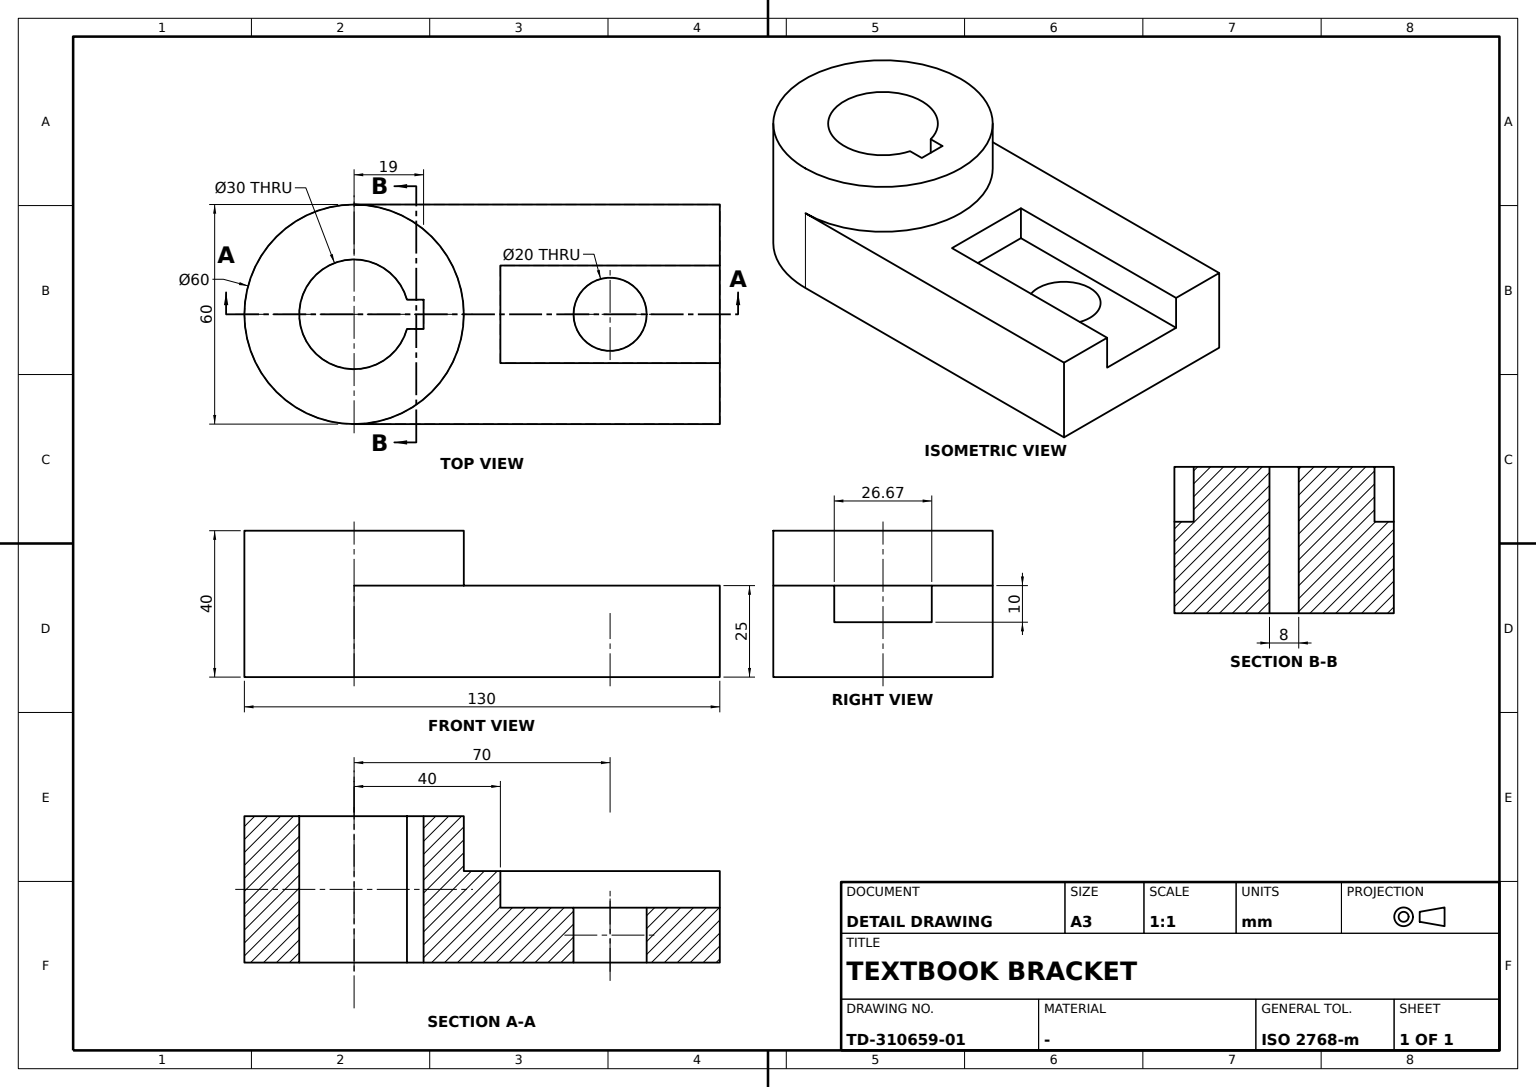
ISO-10303-21;
HEADER;
FILE_DESCRIPTION((''),'2;1');
FILE_NAME('','',(''),(''),'','','');
FILE_SCHEMA(('AUTOMOTIVE_DESIGN'));
ENDSEC;
DATA;
#1=APPLICATION_CONTEXT('');
#2=PRODUCT_CONTEXT('',#1,'mechanical');
#3=PRODUCT('','','',(#2));
#4=PRODUCT_DEFINITION_FORMATION('','',#3);
#5=PRODUCT_DEFINITION_CONTEXT('',#1,'design');
#6=PRODUCT_DEFINITION('','',#4,#5);
#7=PRODUCT_DEFINITION_SHAPE('','',#6);
#8=(LENGTH_UNIT()NAMED_UNIT(*)SI_UNIT(.MILLI.,.METRE.));
#9=(NAMED_UNIT(*)PLANE_ANGLE_UNIT()SI_UNIT($,.RADIAN.));
#10=(NAMED_UNIT(*)SI_UNIT($,.STERADIAN.)SOLID_ANGLE_UNIT());
#11=UNCERTAINTY_MEASURE_WITH_UNIT(LENGTH_MEASURE(1.E-05),#8,'distance_accuracy_value','');
#12=(GEOMETRIC_REPRESENTATION_CONTEXT(3)GLOBAL_UNCERTAINTY_ASSIGNED_CONTEXT((#11))GLOBAL_UNIT_ASSIGNED_CONTEXT((#8,#9,#10))REPRESENTATION_CONTEXT('',''));
#13=CARTESIAN_POINT('',(-4.,14.456832,0.));
#14=VERTEX_POINT('',#13);
#15=CARTESIAN_POINT('',(4.,14.456832,0.));
#16=VERTEX_POINT('',#15);
#17=CARTESIAN_POINT('',(0.,0.,0.));
#18=DIRECTION('',(0.,0.,1.));
#19=DIRECTION('',(0.,1.,0.));
#20=AXIS2_PLACEMENT_3D('',#17,#18,#19);
#21=CIRCLE('',#20,15.);
#22=EDGE_CURVE('',#14,#16,#21,.T.);
#23=ORIENTED_EDGE('',*,*,#22,.T.);
#24=CARTESIAN_POINT('',(4.,19.,0.));
#25=VERTEX_POINT('',#24);
#26=CARTESIAN_POINT('',(4.,16.728416,0.));
#27=VECTOR('',#19,1000.);
#28=LINE('',#26,#27);
#29=EDGE_CURVE('',#16,#25,#28,.T.);
#30=ORIENTED_EDGE('',*,*,#29,.T.);
#31=CARTESIAN_POINT('',(-4.,19.,0.));
#32=VERTEX_POINT('',#31);
#33=CARTESIAN_POINT('',(0.,19.,0.));
#34=DIRECTION('',(-1.,0.,0.));
#35=VECTOR('',#34,1000.);
#36=LINE('',#33,#35);
#37=EDGE_CURVE('',#25,#32,#36,.T.);
#38=ORIENTED_EDGE('',*,*,#37,.T.);
#39=CARTESIAN_POINT('',(-4.,16.728416,0.));
#40=DIRECTION('',(0.,-1.,0.));
#41=VECTOR('',#40,1000.);
#42=LINE('',#39,#41);
#43=EDGE_CURVE('',#32,#14,#42,.T.);
#44=ORIENTED_EDGE('',*,*,#43,.T.);
#45=EDGE_LOOP('',(#23,#30,#38,#44));
#46=FACE_BOUND('',#45,.T.);
#47=CARTESIAN_POINT('',(-30.,100.,0.));
#48=VERTEX_POINT('',#47);
#49=CARTESIAN_POINT('',(-30.,0.,0.));
#50=VERTEX_POINT('',#49);
#51=CARTESIAN_POINT('',(-30.,50.,0.));
#52=LINE('',#51,#41);
#53=EDGE_CURVE('',#48,#50,#52,.T.);
#54=ORIENTED_EDGE('',*,*,#53,.F.);
#55=CARTESIAN_POINT('',(30.,100.,0.));
#56=VERTEX_POINT('',#55);
#57=CARTESIAN_POINT('',(0.,100.,0.));
#58=DIRECTION('',(1.,0.,0.));
#59=VECTOR('',#58,1000.);
#60=LINE('',#57,#59);
#61=EDGE_CURVE('',#48,#56,#60,.T.);
#62=ORIENTED_EDGE('',*,*,#61,.T.);
#63=CARTESIAN_POINT('',(30.,0.,0.));
#64=VERTEX_POINT('',#63);
#65=CARTESIAN_POINT('',(30.,50.,0.));
#66=LINE('',#65,#27);
#67=EDGE_CURVE('',#64,#56,#66,.T.);
#68=ORIENTED_EDGE('',*,*,#67,.F.);
#69=CIRCLE('',#20,30.);
#70=EDGE_CURVE('',#50,#64,#69,.T.);
#71=ORIENTED_EDGE('',*,*,#70,.F.);
#72=EDGE_LOOP('',(#54,#62,#68,#71));
#73=FACE_OUTER_BOUND('',#72,.T.);
#74=CARTESIAN_POINT('',(0.,80.,0.));
#75=VERTEX_POINT('',#74);
#76=CARTESIAN_POINT('',(0.,60.,0.));
#77=VERTEX_POINT('',#76);
#78=CARTESIAN_POINT('',(0.,70.,0.));
#79=AXIS2_PLACEMENT_3D('',#78,#18,#19);
#80=CIRCLE('',#79,10.);
#81=EDGE_CURVE('',#75,#77,#80,.T.);
#82=ORIENTED_EDGE('',*,*,#81,.T.);
#83=EDGE_CURVE('',#77,#75,#80,.T.);
#84=ORIENTED_EDGE('',*,*,#83,.T.);
#85=EDGE_LOOP('',(#82,#84));
#86=FACE_BOUND('',#85,.T.);
#87=PLANE('',#20);
#88=ADVANCED_FACE('',(#46,#73,#86),#87,.F.);
#89=CARTESIAN_POINT('',(-4.,14.456832,40.));
#90=VERTEX_POINT('',#89);
#91=CARTESIAN_POINT('',(4.,14.456832,40.));
#92=VERTEX_POINT('',#91);
#93=CARTESIAN_POINT('',(0.,0.,40.));
#94=AXIS2_PLACEMENT_3D('',#93,#18,#19);
#95=CIRCLE('',#94,15.);
#96=EDGE_CURVE('',#90,#92,#95,.T.);
#97=ORIENTED_EDGE('',*,*,#96,.T.);
#98=CARTESIAN_POINT('',(4.,14.456832,20.));
#99=VECTOR('',#18,1000.);
#100=LINE('',#98,#99);
#101=EDGE_CURVE('',#16,#92,#100,.T.);
#102=ORIENTED_EDGE('',*,*,#101,.F.);
#103=ORIENTED_EDGE('',*,*,#22,.F.);
#104=CARTESIAN_POINT('',(-4.,14.456832,20.));
#105=LINE('',#104,#99);
#106=EDGE_CURVE('',#14,#90,#105,.T.);
#107=ORIENTED_EDGE('',*,*,#106,.T.);
#108=EDGE_LOOP('',(#97,#102,#103,#107));
#109=FACE_OUTER_BOUND('',#108,.T.);
#110=CARTESIAN_POINT('',(0.,0.,20.));
#111=DIRECTION('',(0.,0.,-1.));
#112=AXIS2_PLACEMENT_3D('',#110,#111,#19);
#113=CYLINDRICAL_SURFACE('',#112,15.);
#114=ADVANCED_FACE('',(#109),#113,.F.);
#115=CARTESIAN_POINT('',(-4.,19.,40.));
#116=VERTEX_POINT('',#115);
#117=CARTESIAN_POINT('',(-4.,19.,20.));
#118=LINE('',#117,#99);
#119=EDGE_CURVE('',#32,#116,#118,.T.);
#120=ORIENTED_EDGE('',*,*,#119,.F.);
#121=ORIENTED_EDGE('',*,*,#37,.F.);
#122=CARTESIAN_POINT('',(4.,19.,40.));
#123=VERTEX_POINT('',#122);
#124=CARTESIAN_POINT('',(4.,19.,20.));
#125=LINE('',#124,#99);
#126=EDGE_CURVE('',#25,#123,#125,.T.);
#127=ORIENTED_EDGE('',*,*,#126,.T.);
#128=CARTESIAN_POINT('',(0.,19.,40.));
#129=LINE('',#128,#35);
#130=EDGE_CURVE('',#123,#116,#129,.T.);
#131=ORIENTED_EDGE('',*,*,#130,.T.);
#132=EDGE_LOOP('',(#120,#121,#127,#131));
#133=FACE_OUTER_BOUND('',#132,.T.);
#134=AXIS2_PLACEMENT_3D('',#31,#40,#58);
#135=PLANE('',#134);
#136=ADVANCED_FACE('',(#133),#135,.T.);
#137=CARTESIAN_POINT('',(0.,30.,25.));
#138=VERTEX_POINT('',#137);
#139=CARTESIAN_POINT('',(-30.,0.,25.));
#140=VERTEX_POINT('',#139);
#141=CARTESIAN_POINT('',(0.,0.,25.));
#142=AXIS2_PLACEMENT_3D('',#141,#18,#19);
#143=CIRCLE('',#142,30.);
#144=EDGE_CURVE('',#138,#140,#143,.T.);
#145=ORIENTED_EDGE('',*,*,#144,.F.);
#146=CARTESIAN_POINT('',(30.,0.,25.));
#147=VERTEX_POINT('',#146);
#148=EDGE_CURVE('',#147,#138,#143,.T.);
#149=ORIENTED_EDGE('',*,*,#148,.F.);
#150=CARTESIAN_POINT('',(30.,100.,25.));
#151=VERTEX_POINT('',#150);
#152=CARTESIAN_POINT('',(30.,50.,25.));
#153=LINE('',#152,#27);
#154=EDGE_CURVE('',#147,#151,#153,.T.);
#155=ORIENTED_EDGE('',*,*,#154,.T.);
#156=CARTESIAN_POINT('',(13.332727,100.,25.));
#157=VERTEX_POINT('',#156);
#158=CARTESIAN_POINT('',(21.666364,100.,25.));
#159=LINE('',#158,#59);
#160=EDGE_CURVE('',#157,#151,#159,.T.);
#161=ORIENTED_EDGE('',*,*,#160,.F.);
#162=CARTESIAN_POINT('',(13.332727,40.,25.));
#163=VERTEX_POINT('',#162);
#164=CARTESIAN_POINT('',(13.332727,70.,25.));
#165=LINE('',#164,#41);
#166=EDGE_CURVE('',#157,#163,#165,.T.);
#167=ORIENTED_EDGE('',*,*,#166,.T.);
#168=CARTESIAN_POINT('',(-13.332727,40.,25.));
#169=VERTEX_POINT('',#168);
#170=CARTESIAN_POINT('',(0.,40.,25.));
#171=LINE('',#170,#59);
#172=EDGE_CURVE('',#169,#163,#171,.T.);
#173=ORIENTED_EDGE('',*,*,#172,.F.);
#174=CARTESIAN_POINT('',(-13.332727,100.,25.));
#175=VERTEX_POINT('',#174);
#176=CARTESIAN_POINT('',(-13.332727,70.,25.));
#177=LINE('',#176,#41);
#178=EDGE_CURVE('',#175,#169,#177,.T.);
#179=ORIENTED_EDGE('',*,*,#178,.F.);
#180=CARTESIAN_POINT('',(-30.,100.,25.));
#181=VERTEX_POINT('',#180);
#182=CARTESIAN_POINT('',(-21.666364,100.,25.));
#183=LINE('',#182,#59);
#184=EDGE_CURVE('',#181,#175,#183,.T.);
#185=ORIENTED_EDGE('',*,*,#184,.F.);
#186=CARTESIAN_POINT('',(-30.,50.,25.));
#187=LINE('',#186,#41);
#188=EDGE_CURVE('',#181,#140,#187,.T.);
#189=ORIENTED_EDGE('',*,*,#188,.T.);
#190=EDGE_LOOP('',(#145,#149,#155,#161,#167,#173,#179,#185,#189));
#191=FACE_OUTER_BOUND('',#190,.T.);
#192=PLANE('',#142);
#193=ADVANCED_FACE('',(#191),#192,.T.);
#194=CARTESIAN_POINT('',(0.,80.,15.));
#195=VERTEX_POINT('',#194);
#196=CARTESIAN_POINT('',(0.,60.,15.));
#197=VERTEX_POINT('',#196);
#198=CARTESIAN_POINT('',(0.,70.,15.));
#199=AXIS2_PLACEMENT_3D('',#198,#111,#58);
#200=CIRCLE('',#199,10.);
#201=EDGE_CURVE('',#195,#197,#200,.T.);
#202=ORIENTED_EDGE('',*,*,#201,.T.);
#203=EDGE_CURVE('',#197,#195,#200,.T.);
#204=ORIENTED_EDGE('',*,*,#203,.T.);
#205=EDGE_LOOP('',(#202,#204));
#206=FACE_BOUND('',#205,.T.);
#207=CARTESIAN_POINT('',(-13.332727,100.,15.));
#208=VERTEX_POINT('',#207);
#209=CARTESIAN_POINT('',(-13.332727,40.,15.));
#210=VERTEX_POINT('',#209);
#211=CARTESIAN_POINT('',(-13.332727,70.,15.));
#212=LINE('',#211,#41);
#213=EDGE_CURVE('',#208,#210,#212,.T.);
#214=ORIENTED_EDGE('',*,*,#213,.T.);
#215=CARTESIAN_POINT('',(13.332727,40.,15.));
#216=VERTEX_POINT('',#215);
#217=CARTESIAN_POINT('',(0.,40.,15.));
#218=LINE('',#217,#35);
#219=EDGE_CURVE('',#216,#210,#218,.T.);
#220=ORIENTED_EDGE('',*,*,#219,.F.);
#221=CARTESIAN_POINT('',(13.332727,100.,15.));
#222=VERTEX_POINT('',#221);
#223=CARTESIAN_POINT('',(13.332727,70.,15.));
#224=LINE('',#223,#41);
#225=EDGE_CURVE('',#222,#216,#224,.T.);
#226=ORIENTED_EDGE('',*,*,#225,.F.);
#227=CARTESIAN_POINT('',(0.,100.,15.));
#228=LINE('',#227,#35);
#229=EDGE_CURVE('',#222,#208,#228,.T.);
#230=ORIENTED_EDGE('',*,*,#229,.T.);
#231=EDGE_LOOP('',(#214,#220,#226,#230));
#232=FACE_OUTER_BOUND('',#231,.T.);
#233=AXIS2_PLACEMENT_3D('',#207,#111,#58);
#234=PLANE('',#233);
#235=ADVANCED_FACE('',(#206,#232),#234,.F.);
#236=CARTESIAN_POINT('',(-30.,0.,40.));
#237=VERTEX_POINT('',#236);
#238=CARTESIAN_POINT('',(30.,0.,40.));
#239=VERTEX_POINT('',#238);
#240=CIRCLE('',#94,30.);
#241=EDGE_CURVE('',#237,#239,#240,.T.);
#242=ORIENTED_EDGE('',*,*,#241,.T.);
#243=CARTESIAN_POINT('',(0.,30.,40.));
#244=VERTEX_POINT('',#243);
#245=EDGE_CURVE('',#239,#244,#240,.T.);
#246=ORIENTED_EDGE('',*,*,#245,.T.);
#247=EDGE_CURVE('',#244,#237,#240,.T.);
#248=ORIENTED_EDGE('',*,*,#247,.T.);
#249=EDGE_LOOP('',(#242,#246,#248));
#250=FACE_OUTER_BOUND('',#249,.T.);
#251=CARTESIAN_POINT('',(-4.,16.728416,40.));
#252=LINE('',#251,#41);
#253=EDGE_CURVE('',#116,#90,#252,.T.);
#254=ORIENTED_EDGE('',*,*,#253,.F.);
#255=ORIENTED_EDGE('',*,*,#130,.F.);
#256=CARTESIAN_POINT('',(4.,16.728416,40.));
#257=LINE('',#256,#27);
#258=EDGE_CURVE('',#92,#123,#257,.T.);
#259=ORIENTED_EDGE('',*,*,#258,.F.);
#260=ORIENTED_EDGE('',*,*,#96,.F.);
#261=EDGE_LOOP('',(#254,#255,#259,#260));
#262=FACE_BOUND('',#261,.T.);
#263=PLANE('',#94);
#264=ADVANCED_FACE('',(#250,#262),#263,.T.);
#265=CARTESIAN_POINT('',(-13.332727,40.,20.));
#266=LINE('',#265,#99);
#267=EDGE_CURVE('',#210,#169,#266,.T.);
#268=ORIENTED_EDGE('',*,*,#267,.T.);
#269=ORIENTED_EDGE('',*,*,#172,.T.);
#270=CARTESIAN_POINT('',(13.332727,40.,20.));
#271=VECTOR('',#111,1000.);
#272=LINE('',#270,#271);
#273=EDGE_CURVE('',#163,#216,#272,.T.);
#274=ORIENTED_EDGE('',*,*,#273,.T.);
#275=ORIENTED_EDGE('',*,*,#219,.T.);
#276=EDGE_LOOP('',(#268,#269,#274,#275));
#277=FACE_OUTER_BOUND('',#276,.T.);
#278=CARTESIAN_POINT('',(0.,40.,0.));
#279=AXIS2_PLACEMENT_3D('',#278,#19,#34);
#280=PLANE('',#279);
#281=ADVANCED_FACE('',(#277),#280,.T.);
#282=ORIENTED_EDGE('',*,*,#53,.T.);
#283=CARTESIAN_POINT('',(-30.,0.,12.5));
#284=LINE('',#283,#99);
#285=EDGE_CURVE('',#50,#140,#284,.T.);
#286=ORIENTED_EDGE('',*,*,#285,.T.);
#287=ORIENTED_EDGE('',*,*,#188,.F.);
#288=CARTESIAN_POINT('',(-30.,100.,12.5));
#289=LINE('',#288,#99);
#290=EDGE_CURVE('',#48,#181,#289,.T.);
#291=ORIENTED_EDGE('',*,*,#290,.F.);
#292=EDGE_LOOP('',(#282,#286,#287,#291));
#293=FACE_OUTER_BOUND('',#292,.T.);
#294=AXIS2_PLACEMENT_3D('',#49,#58,#19);
#295=PLANE('',#294);
#296=ADVANCED_FACE('',(#293),#295,.F.);
#297=CARTESIAN_POINT('',(30.,0.,20.));
#298=LINE('',#297,#99);
#299=EDGE_CURVE('',#147,#239,#298,.T.);
#300=ORIENTED_EDGE('',*,*,#299,.F.);
#301=ORIENTED_EDGE('',*,*,#148,.T.);
#302=CARTESIAN_POINT('',(0.,30.,20.));
#303=LINE('',#302,#99);
#304=EDGE_CURVE('',#138,#244,#303,.T.);
#305=ORIENTED_EDGE('',*,*,#304,.T.);
#306=ORIENTED_EDGE('',*,*,#245,.F.);
#307=EDGE_LOOP('',(#300,#301,#305,#306));
#308=FACE_OUTER_BOUND('',#307,.T.);
#309=CYLINDRICAL_SURFACE('',#112,30.);
#310=ADVANCED_FACE('',(#308),#309,.T.);
#311=ORIENTED_EDGE('',*,*,#126,.F.);
#312=ORIENTED_EDGE('',*,*,#29,.F.);
#313=ORIENTED_EDGE('',*,*,#101,.T.);
#314=ORIENTED_EDGE('',*,*,#258,.T.);
#315=EDGE_LOOP('',(#311,#312,#313,#314));
#316=FACE_OUTER_BOUND('',#315,.T.);
#317=AXIS2_PLACEMENT_3D('',#24,#34,#40);
#318=PLANE('',#317);
#319=ADVANCED_FACE('',(#316),#318,.T.);
#320=CARTESIAN_POINT('',(30.,0.,12.5));
#321=LINE('',#320,#99);
#322=EDGE_CURVE('',#64,#147,#321,.T.);
#323=ORIENTED_EDGE('',*,*,#322,.F.);
#324=ORIENTED_EDGE('',*,*,#67,.T.);
#325=CARTESIAN_POINT('',(30.,100.,12.5));
#326=LINE('',#325,#99);
#327=EDGE_CURVE('',#56,#151,#326,.T.);
#328=ORIENTED_EDGE('',*,*,#327,.T.);
#329=ORIENTED_EDGE('',*,*,#154,.F.);
#330=EDGE_LOOP('',(#323,#324,#328,#329));
#331=FACE_OUTER_BOUND('',#330,.T.);
#332=AXIS2_PLACEMENT_3D('',#55,#34,#40);
#333=PLANE('',#332);
#334=ADVANCED_FACE('',(#331),#333,.F.);
#335=CARTESIAN_POINT('',(13.332727,100.,20.));
#336=LINE('',#335,#271);
#337=EDGE_CURVE('',#157,#222,#336,.T.);
#338=ORIENTED_EDGE('',*,*,#337,.F.);
#339=ORIENTED_EDGE('',*,*,#160,.T.);
#340=ORIENTED_EDGE('',*,*,#327,.F.);
#341=ORIENTED_EDGE('',*,*,#61,.F.);
#342=ORIENTED_EDGE('',*,*,#290,.T.);
#343=ORIENTED_EDGE('',*,*,#184,.T.);
#344=CARTESIAN_POINT('',(-13.332727,100.,20.));
#345=LINE('',#344,#99);
#346=EDGE_CURVE('',#208,#175,#345,.T.);
#347=ORIENTED_EDGE('',*,*,#346,.F.);
#348=ORIENTED_EDGE('',*,*,#229,.F.);
#349=EDGE_LOOP('',(#338,#339,#340,#341,#342,#343,#347,#348));
#350=FACE_OUTER_BOUND('',#349,.T.);
#351=CARTESIAN_POINT('',(-20.,100.,0.));
#352=AXIS2_PLACEMENT_3D('',#351,#40,#58);
#353=PLANE('',#352);
#354=ADVANCED_FACE('',(#350),#353,.F.);
#355=CARTESIAN_POINT('',(-30.,0.,20.));
#356=LINE('',#355,#99);
#357=EDGE_CURVE('',#140,#237,#356,.T.);
#358=ORIENTED_EDGE('',*,*,#357,.T.);
#359=ORIENTED_EDGE('',*,*,#247,.F.);
#360=ORIENTED_EDGE('',*,*,#304,.F.);
#361=ORIENTED_EDGE('',*,*,#144,.T.);
#362=EDGE_LOOP('',(#358,#359,#360,#361));
#363=FACE_OUTER_BOUND('',#362,.T.);
#364=ADVANCED_FACE('',(#363),#309,.T.);
#365=ORIENTED_EDGE('',*,*,#203,.F.);
#366=CARTESIAN_POINT('',(0.,60.,12.5));
#367=LINE('',#366,#99);
#368=EDGE_CURVE('',#77,#197,#367,.T.);
#369=ORIENTED_EDGE('',*,*,#368,.F.);
#370=ORIENTED_EDGE('',*,*,#81,.F.);
#371=CARTESIAN_POINT('',(0.,80.,12.5));
#372=LINE('',#371,#99);
#373=EDGE_CURVE('',#75,#195,#372,.T.);
#374=ORIENTED_EDGE('',*,*,#373,.T.);
#375=EDGE_LOOP('',(#365,#369,#370,#374));
#376=FACE_OUTER_BOUND('',#375,.T.);
#377=CARTESIAN_POINT('',(0.,70.,12.5));
#378=AXIS2_PLACEMENT_3D('',#377,#111,#19);
#379=CYLINDRICAL_SURFACE('',#378,10.);
#380=ADVANCED_FACE('',(#376),#379,.F.);
#381=ORIENTED_EDGE('',*,*,#166,.F.);
#382=ORIENTED_EDGE('',*,*,#337,.T.);
#383=ORIENTED_EDGE('',*,*,#225,.T.);
#384=ORIENTED_EDGE('',*,*,#273,.F.);
#385=EDGE_LOOP('',(#381,#382,#383,#384));
#386=FACE_OUTER_BOUND('',#385,.T.);
#387=AXIS2_PLACEMENT_3D('',#221,#58,#18);
#388=PLANE('',#387);
#389=ADVANCED_FACE('',(#386),#388,.F.);
#390=ORIENTED_EDGE('',*,*,#346,.T.);
#391=ORIENTED_EDGE('',*,*,#178,.T.);
#392=ORIENTED_EDGE('',*,*,#267,.F.);
#393=ORIENTED_EDGE('',*,*,#213,.F.);
#394=EDGE_LOOP('',(#390,#391,#392,#393));
#395=FACE_OUTER_BOUND('',#394,.T.);
#396=AXIS2_PLACEMENT_3D('',#174,#34,#111);
#397=PLANE('',#396);
#398=ADVANCED_FACE('',(#395),#397,.F.);
#399=ORIENTED_EDGE('',*,*,#241,.F.);
#400=ORIENTED_EDGE('',*,*,#357,.F.);
#401=ORIENTED_EDGE('',*,*,#285,.F.);
#402=ORIENTED_EDGE('',*,*,#70,.T.);
#403=ORIENTED_EDGE('',*,*,#322,.T.);
#404=ORIENTED_EDGE('',*,*,#299,.T.);
#405=EDGE_LOOP('',(#399,#400,#401,#402,#403,#404));
#406=FACE_OUTER_BOUND('',#405,.T.);
#407=ADVANCED_FACE('',(#406),#309,.T.);
#408=ORIENTED_EDGE('',*,*,#43,.F.);
#409=ORIENTED_EDGE('',*,*,#119,.T.);
#410=ORIENTED_EDGE('',*,*,#253,.T.);
#411=ORIENTED_EDGE('',*,*,#106,.F.);
#412=EDGE_LOOP('',(#408,#409,#410,#411));
#413=FACE_OUTER_BOUND('',#412,.T.);
#414=AXIS2_PLACEMENT_3D('',#13,#58,#19);
#415=PLANE('',#414);
#416=ADVANCED_FACE('',(#413),#415,.T.);
#417=ORIENTED_EDGE('',*,*,#368,.T.);
#418=ORIENTED_EDGE('',*,*,#201,.F.);
#419=ORIENTED_EDGE('',*,*,#373,.F.);
#420=ORIENTED_EDGE('',*,*,#83,.F.);
#421=EDGE_LOOP('',(#417,#418,#419,#420));
#422=FACE_OUTER_BOUND('',#421,.T.);
#423=ADVANCED_FACE('',(#422),#379,.F.);
#424=CLOSED_SHELL('',(#88,#114,#136,#193,#235,#264,#281,#296,#310,#319,#334,#354,#364,#380,#389,#398,#407,#416,#423));
#425=MANIFOLD_SOLID_BREP('',#424);
#426=ADVANCED_BREP_SHAPE_REPRESENTATION('',(#425),#12);
#427=SHAPE_DEFINITION_REPRESENTATION(#7,#426);
ENDSEC;
END-ISO-10303-21;
